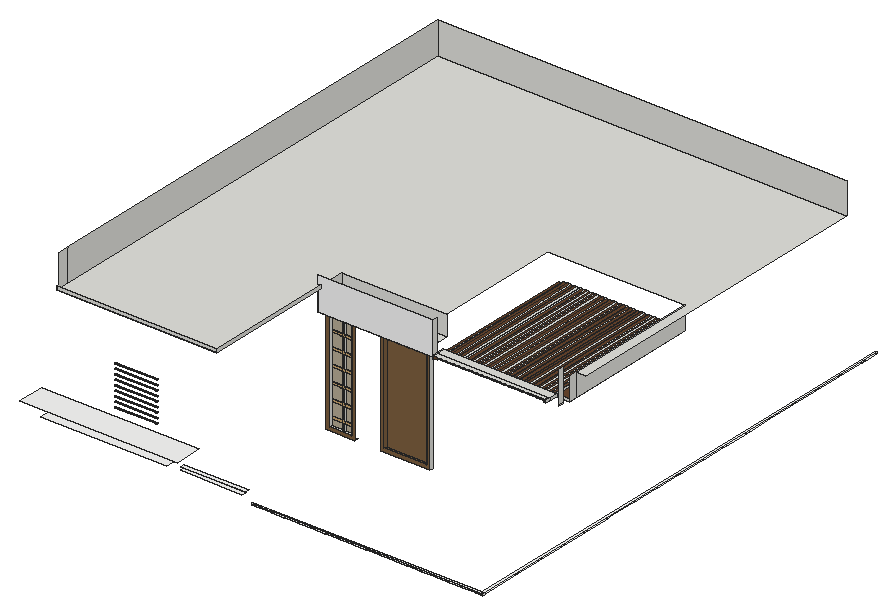
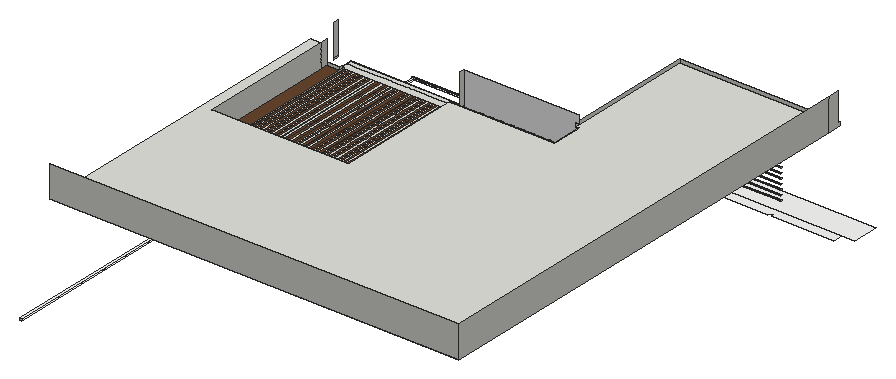
# SketchUp Ruby script. Lengths in inches.
U = 1.inch
M = Sketchup.active_model
def pt(a) = Geom::Point3d.new(a.map { |v| v * U })
def face(e, loops, mat)
  f = e.add_face(loops[0].map { |a| pt(a) })
  loops[1..].each { |l| e.add_face(l.map { |a| pt(a) }).erase! }
  f.material = f.back_material = mat if mat
  f
end
# faces: each face lists its corners as indices into pts; further lists are holes
def faces(e, pts, list, mat = nil) = list.each { |f| face(e, (f[0].is_a?(Array) ? f : [f]).map { |l| l.map { |i| pts[i] } }, mat) }
# xy, xz, yz: faces in a plane at the given z, y or x. An outline is a flat list of corners, or four numbers for a rectangle; further outlines are holes
def ring(l) = l.size == 4 ? [[l[0], l[1]], [l[2], l[1]], [l[2], l[3]], [l[0], l[3]]] : l.each_slice(2).to_a
def flat(e, list, mat, &to3) = list.each { |f| face(e, (f[0].is_a?(Array) ? f : [f]).map { |l| ring(l).map { |u, v| to3.(u, v) } }, mat) }
def xy(e, z, list, mat = nil) = flat(e, list, mat) { |x, y| [x, y, z] }
def xz(e, y, list, mat = nil) = flat(e, list, mat) { |x, z| [x, y, z] }
def yz(e, x, list, mat = nil) = flat(e, list, mat) { |y, z| [x, y, z] }
def lines(e, pts, list) = list.each { |a, b| e.add_line(pt(pts[a]), pt(pts[b])) }
# prism: a flat outline (further loops are holes) pulled along v
def prism(e, loops, v, mat = nil)
  f = face(e, loops, mat); d = Geom::Vector3d.new(v.map { |x| x * U })
  f.pushpull(f.normal.samedirection?(d) ? d.length : -d.length)
end
def box(e, o, s, mat = nil) = prism(e, [[o, [o[0] + s[0], o[1], o[2]], [o[0] + s[0], o[1] + s[1], o[2]], [o[0], o[1] + s[1], o[2]]]], [0, 0, s[2]], mat)
def at(x, y, z, deg = 0) = Geom::Transformation.translation(pt([x, y, z])) * Geom::Transformation.rotation(ORIGIN, Z_AXIS, deg.degrees)
def axes(o, x, y, z) = Geom::Transformation.new([*x, 0, *y, 0, *z, 0, *pt(o).to_a, 1])
def part(name) = M.definitions.add(name)
# library, detail: a bought-in or finely detailed component or shape, given as its bounding box
def library(name, o, s) = part(name).tap { |d| box(d.entities, o, s) }
def detail(e, o, s) = box(e.add_group.entities, o, s)
def put(e, d, t, mat = nil) = e.add_instance(d, t).tap { |i| i.material = mat if mat }
def group(e, t, mat = nil) = e.add_group.tap { |g| g.transformation = t; g.material = mat if mat }.entities
root = M.entities
M.materials.add("CALACATA").color = [248, 248, 247]
M.materials.add("Glass_Mirror_1").color = [185, 173, 151]
M.materials.add("Plywood_01_1K").color = [125, 96, 64]
M.materials.add("Plywood_08_1K").color = [202, 166, 113]
M.materials.add("Wood_Veneer_15_1K").color = [103, 69, 45]
prism(root,[[[75.85,190.16,173.91],[75.85,190.83,173.91],[112.89,190.83,174.06],[112.89,190.16,174.06]]],[0,0,0.46])
box(root,[280.65,439.11,178.23],[34.48,0.67,0.41])
prism(root,[[[75.85,190.16,178.27],[75.85,190.83,178.27],[112.89,190.83,178.41],[112.89,190.16,178.41]]],[0,0,0.46])
box(root,[280.65,439.11,181.59],[34.48,0.67,0.41])
prism(root,[[[75.85,190.16,182.62],[75.85,190.83,182.62],[112.89,190.83,182.76],[112.89,190.16,182.76]]],[0,0,0.46])
box(root,[280.65,439.11,184.94],[34.48,0.67,0.41])
prism(root,[[[75.85,190.16,186.97],[75.85,190.83,186.97],[112.89,190.83,187.11],[112.89,190.16,187.11]]],[0,0,0.46])
box(root,[280.65,439.11,188.29],[34.48,0.67,0.42])
prism(root,[[[75.85,190.16,191.32],[75.85,190.83,191.32],[112.89,190.83,191.47],[112.89,190.16,191.47]]],[0,0,0.46])
box(root,[280.65,439.11,191.65],[34.48,0.67,0.41])
box(root,[280.65,439.11,195],[34.48,0.67,0.42])
prism(root,[[[75.85,190.16,195.68],[75.85,190.83,195.68],[112.89,190.83,195.82],[112.89,190.16,195.82]]],[0,0,0.46])
box(root,[280.65,439.11,198.36],[34.48,0.67,0.41])
prism(root,[[[75.85,190.16,200.03],[75.85,190.83,200.03],[112.89,190.83,200.17],[112.89,190.16,200.17]]],[0,0,0.46])
box(root,[280.65,439.11,201.71],[34.48,0.67,0.41])
prism(root,[[[75.85,190.16,204.38],[75.85,190.83,204.38],[112.89,190.83,204.52],[112.89,190.16,204.52]]],[0,0,0.46])
box(root,[280.65,439.11,205.07],[34.48,0.67,0.41])
prism(root,[[[75.85,190.16,208.73],[75.85,190.83,208.73],[112.89,190.83,208.875],[112.89,190.16,208.875]]],[0,0,0.46])
xy(root,134.12,[[211.23,312.0625,254.75,315.0625]])
xy(root,134.25,[[163.52,312.0625,188.75,315.0625]])
xy(root,137.12,[[214.23,312.0625,251.75,315.0625]],"Plywood_01_1K")
xy(root,137.25,[[166.52,312.0625,185.75,312.0625,185.75,315.0625,178.14,315.0625,178.14,314.0625,176.14,314.0625,176.14,315.0625,166.52,315.0625]])
xy(root,142.91,[[166.52,314.0625,176.14,315.0625],[178.14,314.0625,185.75,315.0625]])
xy(root,144.91,[[166.52,314.0625,176.14,315.0625],[178.14,314.0625,185.75,315.0625]])
xy(root,148.29,[[223.06,178.08,223.57,178.08,223.57,179.51],[205.35,178.14,221.78,179.51],[223.57,178.14,223.57,179.51,408.52,179.51,408.52,178.14,402.875,178.14,402.875,178.65,401.08,178.65,401.08,178.14,390.92,178.14,390.92,178.7,389.13,178.7,389.13,178.14,378.97,178.14,378.97,178.76,377.17,178.76,377.17,178.14,367.01,178.14,367.01,178.82,365.22,178.82,365.22,178.14,355.06,178.14,355.06,178.875,353.27,178.875,353.27,178.14,343.11,178.14,343.11,178.93,341.3125,178.93,341.3125,178.14,331.15,178.14,331.15,178.99,329.36,178.99,329.36,178.14,319.2,178.14,319.2,179.05,317.41,179.05,317.41,178.14,307.25,178.14,307.25,179.11,305.45,179.11,305.45,178.14,295.29,178.14,295.29,179.17,293.5,179.17,293.5,178.14,283.34,178.14,283.34,179.22,281.55,179.22,281.55,178.14,271.39,178.14,271.39,179.28,269.59,179.28,269.59,178.14,259.43,178.14,259.43,179.34,257.64,179.34,257.64,178.14,247.48,178.14,247.48,179.4,245.6875,179.4,245.6875,178.14,235.53,178.14,235.53,179.46,233.73,179.46,233.73,178.14],[233.73,178.14,235.53,179.46],[245.6875,178.14,247.48,179.4],
  [257.64,178.14,259.43,179.34],[269.59,178.14,271.39,179.28],[281.55,178.14,283.34,179.22],[293.5,178.14,295.29,179.17],[305.45,178.14,307.25,179.11],
  [317.41,178.14,319.2,179.05],[329.36,178.14,331.15,178.99],[341.3125,178.14,343.11,178.93],[353.27,178.14,355.06,178.875],[365.22,178.14,367.01,178.82],
  [377.17,178.14,378.97,178.76],[389.13,178.14,390.92,178.7],[401.08,178.14,402.875,178.65],[406.51,179.51,407.89,214.38],[407.94,217.1,407.94,218.18,406.51,218.18],
  [406.51,218.18,406.51,610.73,407.89,610.73,407.89,598.75,407.38,598.75,407.38,594.94,407.89,594.94,407.89,573.38,407.32,573.38,407.32,569.57,407.89,569.57,407.89,548.01,407.26,548.01,407.26,544.2,407.89,544.2,407.89,522.64,407.2,522.64,407.2,518.83,407.89,518.83,407.89,497.27,407.15,497.27,407.15,493.46,407.89,493.46,407.89,471.89,407.09,471.89,407.09,468.09,407.89,468.09,407.89,446.52,407.03,446.52,407.03,442.72,407.89,442.72,407.89,421.15,406.97,421.15,406.97,417.35,407.89,417.35,407.89,395.78,406.92,395.78,406.92,391.98,407.89,391.98,407.89,370.41,406.86,370.41,406.86,366.61,407.89,366.61,407.89,345.04,406.8,345.04,406.8,341.23,407.89,341.23,407.89,319.67,406.74,319.67,406.74,315.86,407.89,315.86,407.89,294.3,406.68,294.3,406.68,290.49,407.89,290.49,407.89,268.93,406.625,268.93,406.625,265.12,407.89,265.12,407.89,243.56,406.57,243.56,406.57,239.75,407.89,239.75,407.89,218.18],[406.57,239.75,407.89,243.56],[406.625,265.12,407.89,268.93],[406.68,290.49,407.89,294.3],[406.74,315.86,407.89,319.67],
  [406.8,341.23,407.89,345.04],[406.86,366.61,407.89,370.41],[406.92,391.98,407.89,395.78],[406.97,417.35,407.89,421.15],[407.03,442.72,407.89,446.52],
  [407.09,468.09,407.89,471.89],[407.15,493.46,407.89,497.27],[407.2,518.83,407.89,522.64],[407.26,544.2,407.89,548.01],[407.32,569.57,407.89,573.38],
  [407.38,594.94,407.89,598.75]],"CALACATA")
xy(root,149.57,[[205.35,178.14,408.52,179.51],[406.51,179.51,407.89,610.73]],"CALACATA")
xy(root,156.52,[[166.52,314.0625,176.14,315.0625],[178.14,314.0625,185.75,315.0625]])
xy(root,158.52,[[166.52,314.0625,176.14,315.0625],[178.14,314.0625,185.75,315.0625]])
xy(root,158.66,[[[148.35,171.04,202.67,174.71],[150.1875,171.76,151,173.13]]],"CALACATA")
xy(root,160,[[28.35,167.73,28.35,191.73,83.14,191.73,83.14,189.73,86.14,189.73,86.14,191.73,139.35,191.73,139.35,167.73]],"CALACATA")
xy(root,161.46,[[148.35,171.04,205.35,174.71]],"CALACATA")
xy(root,166,[[10.35,167.73,148.35,191.73]],"CALACATA")
xy(root,170.13,[[166.52,314.0625,176.14,315.0625],[178.14,314.0625,185.75,315.0625]])
xy(root,172.13,[[166.52,314.0625,176.14,315.0625],[178.14,314.0625,185.75,315.0625]])
xy(root,183.75,[[166.52,314.0625,176.14,315.0625],[178.14,314.0625,185.75,315.0625]])
xy(root,185.75,[[166.52,314.0625,176.14,315.0625],[178.14,314.0625,185.75,315.0625]])
xy(root,197.36,[[166.52,314.0625,176.14,315.0625],[178.14,314.0625,185.75,315.0625]])
xy(root,199.36,[[166.52,314.0625,176.14,315.0625],[178.14,314.0625,185.75,315.0625]])
xy(root,210.97,[[166.52,314.0625,176.14,315.0625],[178.14,314.0625,185.75,315.0625]])
xy(root,212.97,[[166.52,314.0625,176.14,315.0625],[178.14,314.0625,185.75,315.0625]])
xy(root,229,[[166.52,312.0625,166.52,315.0625,176.14,315.0625,176.14,314.0625,178.14,314.0625,178.14,315.0625,185.75,315.0625,185.75,312.0625]])
xy(root,229,[[214.23,312.0625,251.75,315.0625]],"Plywood_01_1K")
xy(root,229.58,[[362.5,302.73,362.5,440.73,375.75,440.73,375.75,314.04,364.23,314.04,364.23,302.73]],"Wood_Veneer_15_1K")
xy(root,229.63,[[264.75,302.73,268.75,440.73]],"Wood_Veneer_15_1K")
xy(root,231.11,[[163.52,302.73,165.52,312.0625],[167.52,302.73,168.46,312.0625],[170.46,302.73,171.4,312.0625],[173.4,302.73,174.34,312.0625],[176.34,302.73,177.28,312.0625],
  [179.28,302.73,180.22,312.0625],[182.22,302.73,183.17,312.0625],[185.17,302.73,186.11,312.0625],[188.11,302.73,189.05,312.0625],[191.05,302.73,191.99,312.0625],
  [193.99,302.73,194.93,312.0625],[196.93,302.73,197.87,312.0625],[199.87,302.73,200.8125,312.0625],[202.8125,302.73,203.75,312.0625],[205.75,302.73,206.69,312.0625],
  [208.69,302.73,209.64,312.0625],[211.64,302.73,212.58,312.0625],[214.58,302.73,215.52,312.0625],[217.52,302.73,218.46,312.0625],[220.46,302.73,221.4,312.0625],
  [223.4,302.73,224.34,312.0625],[226.34,302.73,227.28,312.0625],[229.28,302.73,230.22,312.0625],[232.22,302.73,233.16,312.0625],[235.16,302.73,236.11,312.0625],
  [238.11,302.73,239.05,312.0625],[241.05,302.73,241.99,312.0625],[243.99,302.73,244.93,312.0625],[246.93,302.73,247.87,312.0625],[249.87,302.73,250.8125,312.0625],
  [252.8125,302.73,253.75,312.0625],[268.75,302.73,269.75,440.73],[271.84,302.73,272.84,440.73],[274.9375,302.73,275.9375,440.73],[278.03,302.73,279.03,440.73],
  [281.12,302.73,282.12,440.73],[284.21,302.73,285.21,440.73],[287.3,302.73,288.3,440.73],[290.39,302.73,291.39,440.73],[293.49,302.73,294.49,440.73],
  [296.58,302.73,297.58,440.73],[299.67,302.73,300.67,440.73],[302.76,302.73,303.76,440.73],[305.85,302.73,306.85,440.73],[308.94,302.73,309.94,440.73],
  [312.03,302.73,313.03,440.73],[315.125,302.73,316.125,440.73],[318.22,302.73,319.22,440.73],[321.31,302.73,322.31,440.73],[324.4,302.73,325.4,440.73],
  [327.49,302.73,328.49,440.73],[330.58,302.73,331.58,440.73],[333.68,302.73,334.68,440.73],[336.77,302.73,337.77,440.73],[339.86,302.73,340.86,440.73],
  [342.95,302.73,343.95,440.73],[346.04,302.73,347.04,440.73],[349.13,302.73,350.13,440.73],[352.23,302.73,353.23,440.73],[355.32,302.73,356.32,440.73],
  [358.41,302.73,359.41,440.73],[361.5,302.73,362.5,440.73]])
xy(root,231.11,[[165.52,302.73,167.52,312.0625],[168.46,302.73,170.46,312.0625],[171.4,302.73,173.4,312.0625],[174.34,302.73,176.34,312.0625],[177.28,302.73,179.28,312.0625],
  [180.22,302.73,182.22,312.0625],[183.17,302.73,185.17,312.0625],[186.11,302.73,188.11,312.0625],[189.05,302.73,191.05,312.0625],[191.99,302.73,193.99,312.0625],
  [194.93,302.73,196.93,312.0625],[197.87,302.73,199.87,312.0625],[200.8125,302.73,202.8125,312.0625],[203.75,302.73,205.75,312.0625],[206.69,302.73,208.69,312.0625],
  [209.64,302.73,211.64,312.0625],[212.58,302.73,214.58,312.0625],[215.52,302.73,217.52,312.0625],[218.46,302.73,220.46,312.0625],[221.4,302.73,223.4,312.0625],
  [224.34,302.73,226.34,312.0625],[227.28,302.73,229.28,312.0625],[230.22,302.73,232.22,312.0625],[233.16,302.73,235.16,312.0625],[236.11,302.73,238.11,312.0625],
  [239.05,302.73,241.05,312.0625],[241.99,302.73,243.99,312.0625],[244.93,302.73,246.93,312.0625],[247.87,302.73,249.87,312.0625],[250.8125,302.73,252.8125,312.0625],
  [253.75,302.73,253.75,312.0625,254.75,312.0625,254.75,315.0625,255.75,315.0625,255.75,302.73],[269.75,302.73,271.84,440.73],[272.84,302.73,274.9375,440.73],[275.9375,302.73,278.03,440.73],[279.03,302.73,281.12,440.73],
  [282.12,302.73,284.21,440.73],[285.21,302.73,287.3,440.73],[288.3,302.73,290.39,440.73],[291.39,302.73,293.49,440.73],[294.49,302.73,296.58,440.73],
  [297.58,302.73,299.67,440.73],[300.67,302.73,302.76,440.73],[303.76,302.73,305.85,440.73],[306.85,302.73,308.94,440.73],[309.94,302.73,312.03,440.73],
  [313.03,302.73,315.125,440.73],[316.125,302.73,318.22,440.73],[319.22,302.73,321.31,440.73],[322.31,302.73,324.4,440.73],[325.4,302.73,327.49,440.73],
  [328.49,302.73,330.58,440.73],[331.58,302.73,333.68,440.73],[334.68,302.73,336.77,440.73],[337.77,302.73,339.86,440.73],[340.86,302.73,342.95,440.73],
  [343.95,302.73,346.04,440.73],[347.04,302.73,349.13,440.73],[350.13,302.73,352.23,440.73],[353.23,302.73,355.32,440.73],[356.32,302.73,358.41,440.73],
  [359.41,302.73,361.5,440.73]],"Wood_Veneer_15_1K")
xy(root,232,[[264.75,302.73,364.23,307.15],[264.75,307.15,364.23,314.04],[163.52,312.0625,163.52,320.73,255.75,320.73,255.75,315.0625,254.75,315.0625,254.75,312.0625],[163.52,320.73,255.75,329.73]])
xy(root,250,[[25.35,188.73,25.35,607.49,384.75,607.49,384.75,320.73,375.75,320.73,375.75,440.73,255.75,440.73,255.75,329.73,163.52,329.73,163.52,302.73,166.52,302.73,166.52,188.73]])
xz(root,179.51,[[406.51,148.29,407.89,149.57],[407.89,148.29,408.52,149.57]],"CALACATA")
xz(root,188.73,[[25.35,250,166.52,253]])
xz(root,302.73,[[163.52,231.11,264.75,231.11,264.75,260,163.52,260,163.52,253,166.52,253,166.52,250,163.52,250]],"CALACATA")
xz(root,302.73,[[362.5,229.58,364.23,229.58,364.23,232,264.75,232,264.75,229.63,268.75,229.63,268.75,231.11,362.5,231.11]],"Wood_Veneer_15_1K")
xz(root,312.0625,[[163.52,231.11,188.75,232],[188.75,231.11,211.23,232],[211.23,231.11,254.75,232]])
xz(root,312.0625,[[[211.23,134.12,254.75,231.11],[214.23,137.12,251.75,229]],[[163.52,134.25,188.75,231.11],[166.52,137.25,185.75,229]]],"Plywood_01_1K")
xz(root,314.04,[[364.23,229.58,375.75,232]])
xz(root,314.0625,[[176.14,137.25,178.14,229],[166.52,142.91,176.14,144.91],[178.14,142.91,185.75,144.91],[166.52,156.52,176.14,158.52],[178.14,156.52,185.75,158.52],
  [166.52,170.13,176.14,172.13],[178.14,170.13,185.75,172.13],[166.52,183.75,176.14,185.75],[178.14,183.75,185.75,185.75],[166.52,197.36,176.14,199.36],
  [178.14,197.36,185.75,199.36],[166.52,210.97,176.14,212.97],[178.14,210.97,185.75,212.97]],"Plywood_08_1K")
xz(root,315.0625,[[254.75,231.11,255.75,232]])
xz(root,315.0625,[[166.52,137.25,176.14,142.91],[178.14,137.25,185.75,142.91],[166.52,144.91,176.14,156.52],[178.14,144.91,185.75,156.52],[166.52,158.52,176.14,170.13],
  [178.14,158.52,185.75,170.13],[166.52,172.13,176.14,183.75],[178.14,172.13,185.75,183.75],[166.52,185.75,176.14,197.36],[178.14,185.75,185.75,197.36],
  [166.52,199.36,176.14,210.97],[178.14,199.36,185.75,210.97],[166.52,212.97,176.14,229],[178.14,212.97,185.75,229]],"Glass_Mirror_1")
xz(root,315.0625,[[214.23,137.12,251.75,229]],"Plywood_01_1K")
xz(root,329.73,[[163.52,232,255.75,250]])
xz(root,607.49,[[25.35,250,384.75,278]])
xz(root,610.73,[[406.51,148.29,407.89,149.57]],"CALACATA")
yz(root,25.35,[[188.73,250,188.73,253,190.73,253,190.73,278,200.73,278,200.73,250],[200.73,250,607.49,278]])
yz(root,163.52,[[302.73,231.11,302.73,250,329.73,250,329.73,232,312.0625,232,312.0625,231.11]])
yz(root,166.52,[[312.0625,137.25,315.0625,137.25,315.0625,142.91,314.0625,142.91,314.0625,144.91,315.0625,144.91,315.0625,156.52,314.0625,156.52,314.0625,158.52,315.0625,158.52,315.0625,170.13,314.0625,170.13,314.0625,172.13,315.0625,172.13,315.0625,183.75,314.0625,183.75,314.0625,185.75,315.0625,185.75,315.0625,197.36,314.0625,197.36,314.0625,199.36,315.0625,199.36,315.0625,210.97,314.0625,210.97,314.0625,212.97,315.0625,212.97,315.0625,229,312.0625,229],[188.73,250,302.73,253]])
yz(root,176.14,[[314.0625,137.25,315.0625,142.91],[314.0625,144.91,315.0625,156.52],[314.0625,158.52,315.0625,170.13],[314.0625,172.13,315.0625,183.75],[314.0625,185.75,315.0625,197.36],
  [314.0625,199.36,315.0625,210.97],[314.0625,212.97,315.0625,229]])
yz(root,178.14,[[314.0625,137.25,315.0625,142.91],[314.0625,144.91,315.0625,156.52],[314.0625,158.52,315.0625,170.13],[314.0625,172.13,315.0625,183.75],[314.0625,185.75,315.0625,197.36],
  [314.0625,199.36,315.0625,210.97],[314.0625,212.97,315.0625,229]])
yz(root,185.75,[[312.0625,137.25,312.0625,229,315.0625,229,315.0625,212.97,314.0625,212.97,314.0625,210.97,315.0625,210.97,315.0625,199.36,314.0625,199.36,314.0625,197.36,315.0625,197.36,315.0625,185.75,314.0625,185.75,314.0625,183.75,315.0625,183.75,315.0625,172.13,314.0625,172.13,314.0625,170.13,315.0625,170.13,315.0625,158.52,314.0625,158.52,314.0625,156.52,315.0625,156.52,315.0625,144.91,314.0625,144.91,314.0625,142.91,315.0625,142.91,315.0625,137.25]])
yz(root,205.35,[[178.14,148.29,179.51,149.57]],"CALACATA")
yz(root,214.23,[[312.0625,137.12,315.0625,229]],"Plywood_01_1K")
yz(root,251.75,[[312.0625,137.12,315.0625,229]],"Plywood_01_1K")
yz(root,254.75,[[312.0625,134.12,315.0625,231.11],[312.0625,231.11,315.0625,232]])
yz(root,264.75,[[302.73,229.63,314.04,232],[302.73,232,307.15,260]])
yz(root,268.75,[[302.73,229.63,314.04,231.11],[314.04,229.63,440.73,231.11]])
yz(root,362.5,[[302.73,229.58,314.04,231.11],[314.04,229.58,440.73,231.11]])
yz(root,364.23,[[302.73,229.58,307.15,232],[307.15,229.58,314.04,232]])
yz(root,375.75,[[314.04,229.58,320.73,250],[320.73,229.58,440.73,250],[302.73,231.11,307.15,232],[302.73,232,307.15,260]])
yz(root,408.52,[[178.14,148.29,179.51,149.57]],"CALACATA")
p = [[255.75,329.73,250],[255.75,320.73,250],[375.75,320.73,250],[384.75,321.07,250],[264.75,302.78,232.67],[264.75,302.78,232],
  [156.53,173.13,158.66],[156.53,171.76,158.66],[157.34,171.76,158.66],[157.34,173.13,158.66],[233.73,178.08,148.29],[223.57,178.08,148.29],
  [407.94,239.75,148.29],[407.94,218.18,148.29]]
lines(root,p,[[0,1],[2,3],[4,5],[6,7],[8,9],[10,11],[12,13]])
